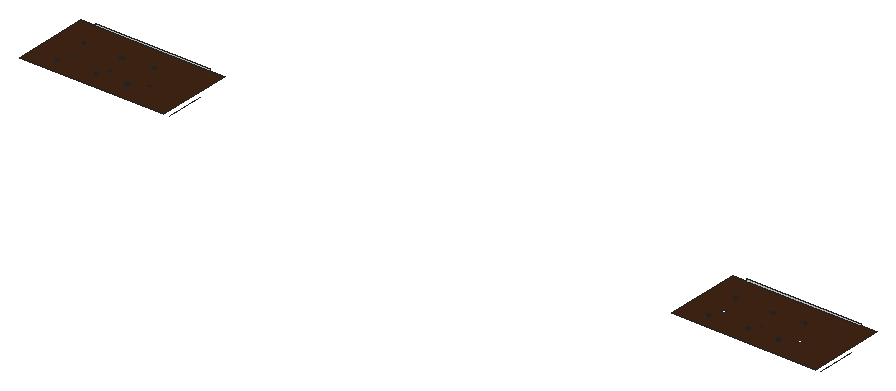
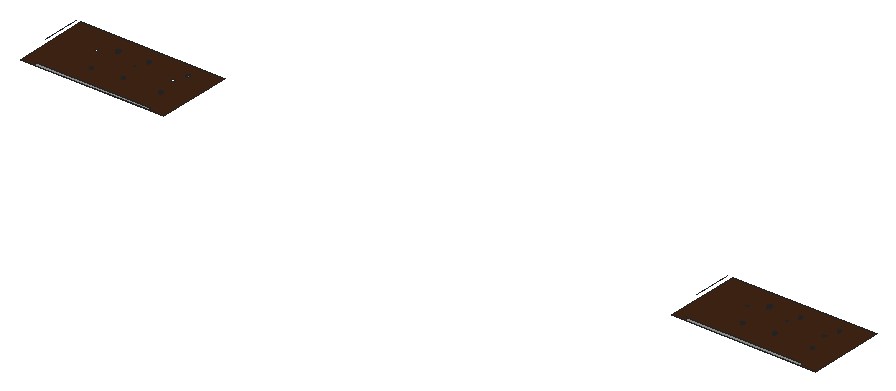
# SketchUp Ruby script. Lengths in inches.
U = 1.inch
M = Sketchup.active_model
def pt(a) = Geom::Point3d.new(a.map { |v| v * U })
def face(e, loops, mat)
  f = e.add_face(loops[0].map { |a| pt(a) })
  loops[1..].each { |l| e.add_face(l.map { |a| pt(a) }).erase! }
  f.material = f.back_material = mat if mat
  f
end
# faces: each face lists its corners as indices into pts; further lists are holes
def faces(e, pts, list, mat = nil) = list.each { |f| face(e, (f[0].is_a?(Array) ? f : [f]).map { |l| l.map { |i| pts[i] } }, mat) }
# xy, xz, yz: faces in a plane at the given z, y or x. An outline is a flat list of corners, or four numbers for a rectangle; further outlines are holes
def ring(l) = l.size == 4 ? [[l[0], l[1]], [l[2], l[1]], [l[2], l[3]], [l[0], l[3]]] : l.each_slice(2).to_a
def flat(e, list, mat, &to3) = list.each { |f| face(e, (f[0].is_a?(Array) ? f : [f]).map { |l| ring(l).map { |u, v| to3.(u, v) } }, mat) }
def xy(e, z, list, mat = nil) = flat(e, list, mat) { |x, y| [x, y, z] }
def xz(e, y, list, mat = nil) = flat(e, list, mat) { |x, z| [x, y, z] }
def yz(e, x, list, mat = nil) = flat(e, list, mat) { |y, z| [x, y, z] }
def lines(e, pts, list) = list.each { |a, b| e.add_line(pt(pts[a]), pt(pts[b])) }
# prism: a flat outline (further loops are holes) pulled along v
def prism(e, loops, v, mat = nil)
  f = face(e, loops, mat); d = Geom::Vector3d.new(v.map { |x| x * U })
  f.pushpull(f.normal.samedirection?(d) ? d.length : -d.length)
end
def box(e, o, s, mat = nil) = prism(e, [[o, [o[0] + s[0], o[1], o[2]], [o[0] + s[0], o[1] + s[1], o[2]], [o[0], o[1] + s[1], o[2]]]], [0, 0, s[2]], mat)
def at(x, y, z, deg = 0) = Geom::Transformation.translation(pt([x, y, z])) * Geom::Transformation.rotation(ORIGIN, Z_AXIS, deg.degrees)
def axes(o, x, y, z) = Geom::Transformation.new([*x, 0, *y, 0, *z, 0, *pt(o).to_a, 1])
def part(name) = M.definitions.add(name)
# library, detail: a bought-in or finely detailed component or shape, given as its bounding box
def library(name, o, s) = part(name).tap { |d| box(d.entities, o, s) }
def detail(e, o, s) = box(e.add_group.entities, o, s)
def put(e, d, t, mat = nil) = e.add_instance(d, t).tap { |i| i.material = mat if mat }
def group(e, t, mat = nil) = e.add_group.tap { |g| g.transformation = t; g.material = mat if mat }.entities
root = M.entities
M.materials.add("[Field Square Tile]").color = [211, 167, 108]
M.materials.add("[Wood Veneer 01]").color = [66, 38, 20]
xy(root,251.5,[[[1990.46,458.5,2184.6,561.05],[2030.6,492.27,2031.39,492.375,2032.13,492.68,2032.76,493.17,2033.25,493.8,2033.56,494.54,2033.66,495.33,2033.56,496.125,2033.25,496.86,2032.76,497.5,2032.13,497.98,2031.39,498.29,2030.6,498.39,2029.81,498.29,2029.07,497.98,2028.43,497.5,2027.95,496.86,2027.64,496.125,2027.54,495.33,2027.64,494.54,2027.95,493.8,2028.43,493.17,2029.07,492.68,2029.81,492.375],[2134.54,492.58,2135.25,492.68,2135.92,492.95,2136.49,493.39,2136.92,493.96,2137.2,494.62,2137.29,495.33,2137.2,496.04,2136.92,496.71,2136.49,497.28,2135.92,497.71,2135.25,497.99,2134.54,498.08,2133.83,497.99,2133.17,497.71,2132.6,497.28,2132.16,496.71,2131.89,496.04,2131.79,495.33,2131.89,494.62,2132.16,493.96,2132.6,493.39,2133.17,492.95,2133.83,492.68],[2081.97,492.77,2082.63,492.86,2083.25,493.11,2083.78,493.52,2084.19,494.05,2084.45,494.67,2084.53,495.33,2084.45,495.99,2084.19,496.61,2083.78,497.14,2083.25,497.55,2082.63,497.81,2081.97,497.89,2081.31,497.81,2080.69,497.55,2080.16,497.14,2079.75,496.61,2079.5,495.99,2079.41,495.33,2079.5,494.67,2079.75,494.05,2080.16,493.52,2080.69,493.11,2081.31,492.86],[2114.7,481.02,2115.33,481.11,2115.92,481.35,2116.42,481.74,2116.81,482.24,2117.05,482.83,2117.13,483.46,2117.05,484.09,2116.81,484.68,2116.42,485.18,2115.92,485.57,2115.33,485.8125,2114.7,485.9,2114.07,485.8125,2113.48,485.57,2112.97,485.18,2112.59,484.68,2112.34,484.09,2112.26,483.46,2112.34,482.83,2112.59,482.24,2112.97,481.74,2113.48,481.35,2114.07,481.11],[2024.3,476.64,2024.78,476.71,2025.24,476.89,2025.625,477.19,2025.92,477.58,2026.11,478.03,2026.17,478.52,2026.11,479,2025.92,479.45,2025.625,479.84,2025.24,480.14,2024.78,480.33,2024.3,480.39,2023.8125,480.33,2023.36,480.14,2022.97,479.84,2022.67,479.45,2022.49,479,2022.42,478.52,2022.49,478.03,2022.67,477.58,2022.97,477.19,2023.36,476.89,2023.8125,476.71],[2024.3,522.58,2024.78,522.64,2025.24,522.83,2025.625,523.13,2025.92,523.52,2026.11,523.97,2026.17,524.45,2026.11,524.94,2025.92,525.39,2025.625,525.78,2025.24,526.08,2024.78,526.27,2024.3,526.33,2023.8125,526.27,2023.36,526.08,2022.97,525.78,2022.67,525.39,2022.49,524.94,2022.42,524.45,2022.49,523.97,2022.67,523.52,2022.97,523.13,2023.36,522.83,2023.8125,522.64],[2074.74,522.58,2075.22,522.64,2075.67,522.83,2076.0625,523.13,2076.36,523.52,2076.55,523.97,2076.61,524.45,2076.55,524.94,2076.36,525.39,2076.0625,525.78,2075.67,526.08,2075.22,526.27,2074.74,526.33,2074.25,526.27,2073.8,526.08,2073.41,525.78,2073.11,525.39,2072.92,524.94,2072.86,524.45,2072.92,523.97,2073.11,523.52,2073.41,523.13,2073.8,522.83,2074.25,522.64],[2074.74,479.77,2075.22,479.83,2075.67,480.02,2076.0625,480.32,2076.36,480.7,2076.55,481.16,2076.61,481.64,2076.55,482.13,2076.36,482.58,2076.0625,482.97,2075.67,483.27,2075.22,483.45,2074.74,483.52,2074.25,483.45,2073.8,483.27,2073.41,482.97,2073.11,482.58,2072.92,482.13,2072.86,481.64,2072.92,481.16,2073.11,480.7,2073.41,480.32,2073.8,480.02,2074.25,479.83],[2114.7,526.75,2115.13,526.8125,2115.54,526.98,2115.89,527.25,2116.16,527.6,2116.33,528,2116.38,528.44,2116.33,528.88,2116.16,529.28,2115.89,529.63,2115.54,529.9,2115.13,530.07,2114.7,530.13,2114.26,530.07,2113.85,529.9,2113.5,529.63,2113.24,529.28,2113.07,528.88,2113.01,528.44,2113.07,528,2113.24,527.6,2113.5,527.25,2113.85,526.98,2114.26,526.8125]],[[2869.21,458.5,3063.35,561.05],[2909.35,492.27,2910.14,492.375,2910.88,492.68,2911.51,493.17,2912,493.8,2912.31,494.54,2912.41,495.33,2912.31,496.125,2912,496.86,2911.51,497.5,2910.88,497.98,2910.14,498.29,2909.35,498.39,2908.56,498.29,2907.82,497.98,2907.18,497.5,2906.7,496.86,2906.39,496.125,2906.29,495.33,2906.39,494.54,2906.7,493.8,2907.18,493.17,2907.82,492.68,2908.56,492.375],[3013.29,492.58,3014,492.68,3014.67,492.95,3015.24,493.39,3015.67,493.96,3015.95,494.62,3016.04,495.33,3015.95,496.04,3015.67,496.71,3015.24,497.28,3014.67,497.71,3014,497.99,3013.29,498.08,3012.58,497.99,3011.92,497.71,3011.35,497.28,3010.91,496.71,3010.64,496.04,3010.54,495.33,3010.64,494.62,3010.91,493.96,3011.35,493.39,3011.92,492.95,3012.58,492.68],[2960.72,492.77,2961.38,492.86,2962,493.11,2962.53,493.52,2962.94,494.05,2963.2,494.67,2963.28,495.33,2963.2,495.99,2962.94,496.61,2962.53,497.14,2962,497.55,2961.38,497.81,2960.72,497.89,2960.06,497.81,2959.44,497.55,2958.91,497.14,2958.5,496.61,2958.25,495.99,2958.16,495.33,2958.25,494.67,2958.5,494.05,2958.91,493.52,2959.44,493.11,2960.06,492.86],[2993.45,481.02,2994.08,481.11,2994.67,481.35,2995.17,481.74,2995.56,482.24,2995.8,482.83,2995.88,483.46,2995.8,484.09,2995.56,484.68,2995.17,485.18,2994.67,485.57,2994.08,485.8125,2993.45,485.9,2992.82,485.8125,2992.23,485.57,2991.72,485.18,2991.34,484.68,2991.09,484.09,2991.01,483.46,2991.09,482.83,2991.34,482.24,2991.72,481.74,2992.23,481.35,2992.82,481.11],[2903.05,522.58,2903.53,522.64,2903.99,522.83,2904.375,523.13,2904.67,523.52,2904.86,523.97,2904.92,524.45,2904.86,524.94,2904.67,525.39,2904.375,525.78,2903.99,526.08,2903.53,526.27,2903.05,526.33,2902.5625,526.27,2902.11,526.08,2901.72,525.78,2901.42,525.39,2901.24,524.94,2901.17,524.45,2901.24,523.97,2901.42,523.52,2901.72,523.13,2902.11,522.83,2902.5625,522.64],[2953.49,522.58,2953.97,522.64,2954.42,522.83,2954.8125,523.13,2955.11,523.52,2955.3,523.97,2955.36,524.45,2955.3,524.94,2955.11,525.39,2954.8125,525.78,2954.42,526.08,2953.97,526.27,2953.49,526.33,2953,526.27,2952.55,526.08,2952.16,525.78,2951.86,525.39,2951.67,524.94,2951.61,524.45,2951.67,523.97,2951.86,523.52,2952.16,523.13,2952.55,522.83,2953,522.64],[2953.49,479.77,2953.97,479.83,2954.42,480.02,2954.8125,480.32,2955.11,480.7,2955.3,481.16,2955.36,481.64,2955.3,482.13,2955.11,482.58,2954.8125,482.97,2954.42,483.27,2953.97,483.45,2953.49,483.52,2953,483.45,2952.55,483.27,2952.16,482.97,2951.86,482.58,2951.67,482.13,2951.61,481.64,2951.67,481.16,2951.86,480.7,2952.16,480.32,2952.55,480.02,2953,479.83],[2903.05,476.64,2903.53,476.71,2903.99,476.89,2904.375,477.19,2904.67,477.58,2904.86,478.03,2904.92,478.52,2904.86,479,2904.67,479.45,2904.375,479.84,2903.99,480.14,2903.53,480.33,2903.05,480.39,2902.5625,480.33,2902.11,480.14,2901.72,479.84,2901.42,479.45,2901.24,479,2901.17,478.52,2901.24,478.03,2901.42,477.58,2901.72,477.19,2902.11,476.89,2902.5625,476.71],[2993.45,526.75,2993.88,526.8125,2994.29,526.98,2994.64,527.25,2994.91,527.6,2995.08,528,2995.13,528.44,2995.08,528.88,2994.91,529.28,2994.64,529.63,2994.29,529.9,2993.88,530.07,2993.45,530.13,2993.01,530.07,2992.6,529.9,2992.25,529.63,2991.99,529.28,2991.82,528.88,2991.76,528.44,2991.82,528,2991.99,527.6,2992.25,527.25,2992.6,526.98,2993.01,526.8125]]],"[Wood Veneer 01]")
xz(root,561.05,[[2010.28,251.5,2010.34,254.5],[2010.34,251.5,2164.35,254.5],[2889.03,251.5,2889.09,254.5],[2889.09,251.5,3043.1,254.5]])
p = [[2024.3,476.64,251.5],[2023.8125,476.71,251.5],[2023.8125,476.71,252.5],[2024.3,476.64,252.5],[2024.78,476.71,251.5],[2024.78,476.71,252.5],
  [2903.05,476.64,251.5],[2902.5625,476.71,251.5],[2902.5625,476.71,252.5],[2903.05,476.64,252.5],[2903.53,476.71,251.5],[2903.53,476.71,252.5],
  [2023.36,476.89,251.5],[2023.36,476.89,252.5],[2025.24,476.89,251.5],[2025.24,476.89,252.5],[2902.11,476.89,251.5],[2902.11,476.89,252.5],
  [2903.99,476.89,251.5],[2903.99,476.89,252.5],[2022.97,477.19,251.5],[2022.97,477.19,252.5],[2025.625,477.19,251.5],[2025.625,477.19,252.5],
  [2901.72,477.19,251.5],[2901.72,477.19,252.5],[2904.375,477.19,251.5],[2904.375,477.19,252.5],[2022.67,477.58,251.5],[2022.67,477.58,252.5],
  [2025.92,477.58,251.5],[2025.92,477.58,252.5],[2901.42,477.58,251.5],[2901.42,477.58,252.5],[2904.67,477.58,251.5],[2904.67,477.58,252.5],
  [2022.49,478.03,251.5],[2022.49,478.03,252.5],[2026.11,478.03,251.5],[2026.11,478.03,252.5],[2901.24,478.03,251.5],[2901.24,478.03,252.5],
  [2904.86,478.03,251.5],[2904.86,478.03,252.5],[2022.42,478.52,251.5],[2022.42,478.52,252.5],[2026.17,478.52,251.5],[2026.17,478.52,252.5],
  [2901.17,478.52,251.5],[2901.17,478.52,252.5],[2904.92,478.52,251.5],[2904.92,478.52,252.5],[2022.49,479,251.5],[2022.49,479,252.5],
  [2026.11,479,251.5],[2026.11,479,252.5],[2901.24,479,251.5],[2901.24,479,252.5],[2904.86,479,251.5],[2904.86,479,252.5],
  [2022.67,479.45,251.5],[2022.67,479.45,252.5],[2025.92,479.45,251.5],[2025.92,479.45,252.5],[2901.42,479.45,251.5],[2901.42,479.45,252.5],
  [2904.67,479.45,251.5],[2904.67,479.45,252.5],[2022.97,479.84,251.5],[2022.97,479.84,252.5],[2025.625,479.84,251.5],[2025.625,479.84,252.5],
  [2901.72,479.84,251.5],[2901.72,479.84,252.5],[2904.375,479.84,251.5],[2904.375,479.84,252.5],[2023.36,480.14,251.5],[2023.36,480.14,252.5],
  [2025.24,480.14,251.5],[2025.24,480.14,252.5],[2074.25,479.83,251.5],[2073.8,480.02,251.5],[2073.8,480.02,252.5],[2074.25,479.83,252.5],
  [2074.74,479.77,251.5],[2074.74,479.77,252.5],[2075.22,479.83,251.5],[2075.22,479.83,252.5],[2075.67,480.02,251.5],[2075.67,480.02,252.5],
  [2902.11,480.14,251.5],[2902.11,480.14,252.5],[2903.99,480.14,251.5],[2903.99,480.14,252.5],[2953,479.83,251.5],[2952.55,480.02,251.5],
  [2952.55,480.02,252.5],[2953,479.83,252.5],[2953.49,479.77,251.5],[2953.49,479.77,252.5],[2953.97,479.83,251.5],[2953.97,479.83,252.5],
  [2954.42,480.02,251.5],[2954.42,480.02,252.5],[2073.41,480.32,251.5],[2073.41,480.32,252.5],[2076.0625,480.32,251.5],[2076.0625,480.32,252.5],
  [2952.16,480.32,251.5],[2952.16,480.32,252.5],[2954.8125,480.32,251.5],[2954.8125,480.32,252.5],[2023.8125,480.33,251.5],[2023.8125,480.33,252.5],
  [2024.78,480.33,251.5],[2024.78,480.33,252.5],[2902.5625,480.33,251.5],[2902.5625,480.33,252.5],[2903.53,480.33,251.5],[2903.53,480.33,252.5],
  [2024.3,480.39,251.5],[2024.3,480.39,252.5],[2073.11,480.7,251.5],[2073.11,480.7,252.5],[2076.36,480.7,251.5],[2076.36,480.7,252.5],
  [2903.05,480.39,251.5],[2903.05,480.39,252.5],[2951.86,480.7,251.5],[2951.86,480.7,252.5],[2955.11,480.7,251.5],[2955.11,480.7,252.5],
  [2072.92,481.16,251.5],[2072.92,481.16,252.5],[2076.55,481.16,251.5],[2076.55,481.16,252.5],[2951.67,481.16,251.5],[2951.67,481.16,252.5],
  [2955.3,481.16,251.5],[2955.3,481.16,252.5],[2114.7,481.02,251.5],[2114.07,481.11,251.5],[2114.07,481.11,252.5625],[2114.7,481.02,252.5625],
  [2115.33,481.11,251.5],[2115.33,481.11,252.5625],[2993.45,481.02,251.5],[2992.82,481.11,251.5],[2992.82,481.11,252.5625],[2993.45,481.02,252.5625],
  [2994.08,481.11,251.5],[2994.08,481.11,252.5625],[2113.48,481.35,251.5],[2113.48,481.35,252.5625],[2115.92,481.35,251.5],[2115.92,481.35,252.5625],
  [2992.23,481.35,251.5],[2992.23,481.35,252.5625],[2994.67,481.35,251.5],[2994.67,481.35,252.5625],[2072.86,481.64,251.5],[2072.86,481.64,252.5],
  [2076.61,481.64,251.5],[2076.61,481.64,252.5],[2951.61,481.64,251.5],[2951.61,481.64,252.5],[2955.36,481.64,251.5],[2955.36,481.64,252.5],
  [2112.97,481.74,251.5],[2112.97,481.74,252.5625],[2116.42,481.74,251.5],[2116.42,481.74,252.5625],[2991.72,481.74,251.5],[2991.72,481.74,252.5625],
  [2995.17,481.74,251.5],[2995.17,481.74,252.5625],[2072.92,482.13,251.5],[2072.92,482.13,252.5],[2076.55,482.13,251.5],[2076.55,482.13,252.5],
  [2951.67,482.13,251.5],[2951.67,482.13,252.5],[2955.3,482.13,251.5],[2955.3,482.13,252.5],[2112.59,482.24,251.5],[2112.59,482.24,252.5625],
  [2116.81,482.24,251.5],[2116.81,482.24,252.5625],[2991.34,482.24,251.5],[2991.34,482.24,252.5625],[2995.56,482.24,251.5],[2995.56,482.24,252.5625],
  [2073.11,482.58,251.5],[2073.11,482.58,252.5],[2076.36,482.58,251.5],[2076.36,482.58,252.5],[2951.86,482.58,251.5],[2951.86,482.58,252.5],
  [2955.11,482.58,251.5],[2955.11,482.58,252.5],[2112.34,482.83,251.5],[2112.34,482.83,252.5625],[2117.05,482.83,251.5],[2117.05,482.83,252.5625],
  [2991.09,482.83,251.5],[2991.09,482.83,252.5625],[2995.8,482.83,251.5],[2995.8,482.83,252.5625],[2073.41,482.97,251.5],[2073.41,482.97,252.5],
  [2076.0625,482.97,251.5],[2076.0625,482.97,252.5],[2952.16,482.97,251.5],[2952.16,482.97,252.5],[2954.8125,482.97,251.5],[2954.8125,482.97,252.5],
  [2112.26,483.46,251.5],[2112.26,483.46,252.5625],[2117.13,483.46,251.5],[2117.13,483.46,252.5625],[2991.01,483.46,251.5],[2991.01,483.46,252.5625],
  [2995.88,483.46,251.5],[2995.88,483.46,252.5625],[2073.8,483.27,251.5],[2073.8,483.27,252.5],[2075.67,483.27,251.5],[2075.67,483.27,252.5],
  [2952.55,483.27,251.5],[2952.55,483.27,252.5],[2954.42,483.27,251.5],[2954.42,483.27,252.5],[2074.25,483.45,251.5],[2074.25,483.45,252.5],
  [2075.22,483.45,251.5],[2075.22,483.45,252.5],[2953,483.45,251.5],[2953,483.45,252.5],[2953.97,483.45,251.5],[2953.97,483.45,252.5],
  [2074.74,483.52,251.5],[2074.74,483.52,252.5],[2112.34,484.09,251.5],[2112.34,484.09,252.5625],[2117.05,484.09,251.5],[2117.05,484.09,252.5625],
  [2953.49,483.52,251.5],[2953.49,483.52,252.5],[2991.09,484.09,251.5],[2991.09,484.09,252.5625],[2995.8,484.09,251.5],[2995.8,484.09,252.5625],
  [2112.59,484.68,251.5],[2112.59,484.68,252.5625],[2116.81,484.68,251.5],[2116.81,484.68,252.5625],[2991.34,484.68,251.5],[2991.34,484.68,252.5625],
  [2995.56,484.68,251.5],[2995.56,484.68,252.5625],[2112.97,485.18,251.5],[2112.97,485.18,252.5625],[2116.42,485.18,251.5],[2116.42,485.18,252.5625],
  [2991.72,485.18,251.5],[2991.72,485.18,252.5625],[2995.17,485.18,251.5],[2995.17,485.18,252.5625],[2113.48,485.57,251.5],[2113.48,485.57,252.5625],
  [2115.92,485.57,251.5],[2115.92,485.57,252.5625],[2992.23,485.57,251.5],[2992.23,485.57,252.5625],[2994.67,485.57,251.5],[2994.67,485.57,252.5625],
  [2114.07,485.8125,251.5],[2114.07,485.8125,252.5625],[2115.33,485.8125,251.5],[2115.33,485.8125,252.5625],[2992.82,485.8125,251.5],[2992.82,485.8125,252.5625],
  [2994.08,485.8125,251.5],[2994.08,485.8125,252.5625],[2114.7,485.9,251.5],[2114.7,485.9,252.5625],[2993.45,485.9,251.5],[2993.45,485.9,252.5625],
  [2023.8125,522.64,251.5],[2023.36,522.83,251.5],[2023.36,522.83,252.5],[2023.8125,522.64,252.5],[2024.3,522.58,251.5],[2024.3,522.58,252.5],
  [2024.78,522.64,251.5],[2024.78,522.64,252.5],[2025.24,522.83,251.5],[2025.24,522.83,252.5],[2074.25,522.64,251.5],[2073.8,522.83,251.5],
  [2073.8,522.83,252.5],[2074.25,522.64,252.5],[2074.74,522.58,251.5],[2074.74,522.58,252.5],[2075.22,522.64,251.5],[2075.22,522.64,252.5],
  [2075.67,522.83,251.5],[2075.67,522.83,252.5],[2902.5625,522.64,251.5],[2902.11,522.83,251.5],[2902.11,522.83,252.5],[2902.5625,522.64,252.5],
  [2903.05,522.58,251.5],[2903.05,522.58,252.5],[2903.53,522.64,251.5],[2903.53,522.64,252.5],[2903.99,522.83,251.5],[2903.99,522.83,252.5],
  [2953,522.64,251.5],[2952.55,522.83,251.5],[2952.55,522.83,252.5],[2953,522.64,252.5],[2953.49,522.58,251.5],[2953.49,522.58,252.5],
  [2953.97,522.64,251.5],[2953.97,522.64,252.5],[2954.42,522.83,251.5],[2954.42,522.83,252.5],[2022.97,523.13,251.5],[2022.97,523.13,252.5],
  [2025.625,523.13,251.5],[2025.625,523.13,252.5],[2073.41,523.13,251.5],[2073.41,523.13,252.5],[2076.0625,523.13,251.5],[2076.0625,523.13,252.5],
  [2901.72,523.13,251.5],[2901.72,523.13,252.5],[2904.375,523.13,251.5],[2904.375,523.13,252.5],[2952.16,523.13,251.5],[2952.16,523.13,252.5],
  [2954.8125,523.13,251.5],[2954.8125,523.13,252.5],[2022.67,523.52,251.5],[2022.67,523.52,252.5],[2025.92,523.52,251.5],[2025.92,523.52,252.5],
  [2073.11,523.52,251.5],[2073.11,523.52,252.5],[2076.36,523.52,251.5],[2076.36,523.52,252.5],[2901.42,523.52,251.5],[2901.42,523.52,252.5],
  [2904.67,523.52,251.5],[2904.67,523.52,252.5],[2951.86,523.52,251.5],[2951.86,523.52,252.5],[2955.11,523.52,251.5],[2955.11,523.52,252.5],
  [2022.49,523.97,251.5],[2022.49,523.97,252.5],[2026.11,523.97,251.5],[2026.11,523.97,252.5],[2072.92,523.97,251.5],[2072.92,523.97,252.5],
  [2076.55,523.97,251.5],[2076.55,523.97,252.5],[2901.24,523.97,251.5],[2901.24,523.97,252.5],[2904.86,523.97,251.5],[2904.86,523.97,252.5],
  [2951.67,523.97,251.5],[2951.67,523.97,252.5],[2955.3,523.97,251.5],[2955.3,523.97,252.5],[2022.42,524.45,251.5],[2022.42,524.45,252.5],
  [2026.17,524.45,251.5],[2026.17,524.45,252.5],[2072.86,524.45,251.5],[2072.86,524.45,252.5],[2076.61,524.45,251.5],[2076.61,524.45,252.5],
  [2901.17,524.45,251.5],[2901.17,524.45,252.5],[2904.92,524.45,251.5],[2904.92,524.45,252.5],[2951.61,524.45,251.5],[2951.61,524.45,252.5],
  [2955.36,524.45,251.5],[2955.36,524.45,252.5],[2022.49,524.94,251.5],[2022.49,524.94,252.5],[2026.11,524.94,251.5],[2026.11,524.94,252.5],
  [2072.92,524.94,251.5],[2072.92,524.94,252.5],[2076.55,524.94,251.5],[2076.55,524.94,252.5],[2901.24,524.94,251.5],[2901.24,524.94,252.5],
  [2904.86,524.94,251.5],[2904.86,524.94,252.5],[2951.67,524.94,251.5],[2951.67,524.94,252.5],[2955.3,524.94,251.5],[2955.3,524.94,252.5],
  [2022.67,525.39,251.5],[2022.67,525.39,252.5],[2025.92,525.39,251.5],[2025.92,525.39,252.5],[2073.11,525.39,251.5],[2073.11,525.39,252.5],
  [2076.36,525.39,251.5],[2076.36,525.39,252.5],[2901.42,525.39,251.5],[2901.42,525.39,252.5],[2904.67,525.39,251.5],[2904.67,525.39,252.5],
  [2951.86,525.39,251.5],[2951.86,525.39,252.5],[2955.11,525.39,251.5],[2955.11,525.39,252.5],[2022.97,525.78,251.5],[2022.97,525.78,252.5],
  [2025.625,525.78,251.5],[2025.625,525.78,252.5],[2073.41,525.78,251.5],[2073.41,525.78,252.5],[2076.0625,525.78,251.5],[2076.0625,525.78,252.5],
  [2901.72,525.78,251.5],[2901.72,525.78,252.5],[2904.375,525.78,251.5],[2904.375,525.78,252.5],[2952.16,525.78,251.5],[2952.16,525.78,252.5],
  [2954.8125,525.78,251.5],[2954.8125,525.78,252.5],[2023.36,526.08,251.5],[2023.36,526.08,252.5],[2025.24,526.08,251.5],[2025.24,526.08,252.5],
  [2073.8,526.08,251.5],[2073.8,526.08,252.5],[2075.67,526.08,251.5],[2075.67,526.08,252.5],[2902.11,526.08,251.5],[2902.11,526.08,252.5],
  [2903.99,526.08,251.5],[2903.99,526.08,252.5],[2952.55,526.08,251.5],[2952.55,526.08,252.5],[2954.42,526.08,251.5],[2954.42,526.08,252.5],
  [2023.8125,526.27,251.5],[2023.8125,526.27,252.5],[2024.78,526.27,251.5],[2024.78,526.27,252.5],[2074.25,526.27,251.5],[2074.25,526.27,252.5],
  [2075.22,526.27,251.5],[2075.22,526.27,252.5],[2902.5625,526.27,251.5],[2902.5625,526.27,252.5],[2903.53,526.27,251.5],[2903.53,526.27,252.5],
  [2953,526.27,251.5],[2953,526.27,252.5],[2953.97,526.27,251.5],[2953.97,526.27,252.5],[2024.3,526.33,251.5],[2024.3,526.33,252.5],
  [2074.74,526.33,251.5],[2074.74,526.33,252.5],[2903.05,526.33,251.5],[2903.05,526.33,252.5],[2953.49,526.33,251.5],[2953.49,526.33,252.5],
  [2114.26,526.8125,251.5],[2113.85,526.98,251.5],[2113.85,526.98,252.4375],[2114.26,526.8125,252.4375],[2114.7,526.75,251.5],[2114.7,526.75,252.4375],
  [2115.13,526.8125,251.5],[2115.13,526.8125,252.4375],[2115.54,526.98,251.5],[2115.54,526.98,252.4375],[2993.01,526.8125,251.5],[2992.6,526.98,251.5],
  [2992.6,526.98,252.4375],[2993.01,526.8125,252.4375],[2993.45,526.75,251.5],[2993.45,526.75,252.4375],[2993.88,526.8125,251.5],[2993.88,526.8125,252.4375],
  [2994.29,526.98,251.5],[2994.29,526.98,252.4375],[2113.5,527.25,251.5],[2113.5,527.25,252.4375],[2115.89,527.25,251.5],[2115.89,527.25,252.4375],
  [2992.25,527.25,251.5],[2992.25,527.25,252.4375],[2994.64,527.25,251.5],[2994.64,527.25,252.4375],[2113.24,527.6,251.5],[2113.24,527.6,252.4375],
  [2116.16,527.6,251.5],[2116.16,527.6,252.4375],[2991.99,527.6,251.5],[2991.99,527.6,252.4375],[2994.91,527.6,251.5],[2994.91,527.6,252.4375],
  [2113.07,528,251.5],[2113.07,528,252.4375],[2116.33,528,251.5],[2116.33,528,252.4375],[2991.82,528,251.5],[2991.82,528,252.4375],
  [2995.08,528,251.5],[2995.08,528,252.4375],[2113.01,528.44,251.5],[2113.01,528.44,252.4375],[2116.38,528.44,251.5],[2116.38,528.44,252.4375],
  [2991.76,528.44,251.5],[2991.76,528.44,252.4375],[2995.13,528.44,251.5],[2995.13,528.44,252.4375],[2113.07,528.88,251.5],[2113.07,528.88,252.4375],
  [2116.33,528.88,251.5],[2116.33,528.88,252.4375],[2991.82,528.88,251.5],[2991.82,528.88,252.4375],[2995.08,528.88,251.5],[2995.08,528.88,252.4375],
  [2113.24,529.28,251.5],[2113.24,529.28,252.4375],[2116.16,529.28,251.5],[2116.16,529.28,252.4375],[2991.99,529.28,251.5],[2991.99,529.28,252.4375],
  [2994.91,529.28,251.5],[2994.91,529.28,252.4375],[2113.5,529.63,251.5],[2113.5,529.63,252.4375],[2115.89,529.63,251.5],[2115.89,529.63,252.4375],
  [2992.25,529.63,251.5],[2992.25,529.63,252.4375],[2994.64,529.63,251.5],[2994.64,529.63,252.4375],[2113.85,529.9,251.5],[2113.85,529.9,252.4375],
  [2115.54,529.9,251.5],[2115.54,529.9,252.4375],[2992.6,529.9,251.5],[2992.6,529.9,252.4375],[2994.29,529.9,251.5],[2994.29,529.9,252.4375],
  [2114.26,530.07,251.5],[2114.26,530.07,252.4375],[2115.13,530.07,251.5],[2115.13,530.07,252.4375],[2993.01,530.07,251.5],[2993.01,530.07,252.4375],
  [2993.88,530.07,251.5],[2993.88,530.07,252.4375],[2114.7,530.13,251.5],[2114.7,530.13,252.4375],[2993.45,530.13,251.5],[2993.45,530.13,252.4375],
  [2191.47,511.08,251.5],[2191.47,458.5,251.5],[3070.22,511.08,251.5],[3070.22,458.5,251.5]]
faces(root,p,[[0,1,2,3],[4,0,3,5],[6,7,8,9],[10,6,9,11],[1,12,13,2],[14,4,5,15],[7,16,17,8],[18,10,11,19],
  [12,20,21,13],[22,14,15,23],[16,24,25,17],[26,18,19,27],[20,28,29,21],[30,22,23,31],[24,32,33,25],[34,26,27,35],
  [28,36,37,29],[38,30,31,39],[32,40,41,33],[42,34,35,43],[36,44,45,37],[46,38,39,47],[40,48,49,41],[50,42,43,51],
  [44,52,53,45],[54,46,47,55],[48,56,57,49],[58,50,51,59],[52,60,61,53],[62,54,55,63],[56,64,65,57],[66,58,59,67],
  [60,68,69,61],[70,62,63,71],[64,72,73,65],[74,66,67,75],[68,76,77,69],[78,70,71,79],[80,81,82,83],[84,80,83,85],
  [86,84,85,87],[88,86,87,89],[72,90,91,73],[92,74,75,93],[94,95,96,97],[98,94,97,99],[100,98,99,101],[102,100,101,103],
  [81,104,105,82],[106,88,89,107],[95,108,109,96],[110,102,103,111],[76,112,113,77],[114,78,79,115],[90,116,117,91],[118,92,93,119],
  [112,120,121,113],[120,114,115,121],[104,122,123,105],[124,106,107,125],[116,126,127,117],[126,118,119,127],[108,128,129,109],[130,110,111,131],
  [122,132,133,123],[134,124,125,135],[128,136,137,129],[138,130,131,139],[140,141,142,143],[144,140,143,145],[146,147,148,149],[150,146,149,151],
  [141,152,153,142],[154,144,145,155],[147,156,157,148],[158,150,151,159],[132,160,161,133],[162,134,135,163],[136,164,165,137],[166,138,139,167],
  [152,168,169,153],[170,154,155,171],[156,172,173,157],[174,158,159,175],[160,176,177,161],[178,162,163,179],[164,180,181,165],[182,166,167,183],
  [168,184,185,169],[186,170,171,187],[172,188,189,173],[190,174,175,191],[176,192,193,177],[194,178,179,195],[180,196,197,181],[198,182,183,199],
  [184,200,201,185],[202,186,187,203],[188,204,205,189],[206,190,191,207],[192,208,209,193],[210,194,195,211],[196,212,213,197],[214,198,199,215],
  [200,216,217,201],[218,202,203,219],[204,220,221,205],[222,206,207,223],[208,224,225,209],[226,210,211,227],[212,228,229,213],[230,214,215,231],
  [224,232,233,225],[234,226,227,235],[228,236,237,229],[238,230,231,239],[232,240,241,233],[240,234,235,241],[216,242,243,217],[244,218,219,245],
  [236,246,247,237],[246,238,239,247],[220,248,249,221],[250,222,223,251],[242,252,253,243],[254,244,245,255],[248,256,257,249],[258,250,251,259],
  [252,260,261,253],[262,254,255,263],[256,264,265,257],[266,258,259,267],[260,268,269,261],[270,262,263,271],[264,272,273,265],[274,266,267,275],
  [268,276,277,269],[278,270,271,279],[272,280,281,273],[282,274,275,283],[276,284,285,277],[284,278,279,285],[280,286,287,281],[286,282,283,287],
  [288,289,290,291],[292,288,291,293],[294,292,293,295],[296,294,295,297],[298,299,300,301],[302,298,301,303],[304,302,303,305],[306,304,305,307],
  [308,309,310,311],[312,308,311,313],[314,312,313,315],[316,314,315,317],[318,319,320,321],[322,318,321,323],[324,322,323,325],[326,324,325,327],
  [289,328,329,290],[330,296,297,331],[299,332,333,300],[334,306,307,335],[309,336,337,310],[338,316,317,339],[319,340,341,320],[342,326,327,343],
  [328,344,345,329],[346,330,331,347],[332,348,349,333],[350,334,335,351],[336,352,353,337],[354,338,339,355],[340,356,357,341],[358,342,343,359],
  [344,360,361,345],[362,346,347,363],[348,364,365,349],[366,350,351,367],[352,368,369,353],[370,354,355,371],[356,372,373,357],[374,358,359,375],
  [360,376,377,361],[378,362,363,379],[364,380,381,365],[382,366,367,383],[368,384,385,369],[386,370,371,387],[372,388,389,373],[390,374,375,391],
  [376,392,393,377],[394,378,379,395],[380,396,397,381],[398,382,383,399],[384,400,401,385],[402,386,387,403],[388,404,405,389],[406,390,391,407],
  [392,408,409,393],[410,394,395,411],[396,412,413,397],[414,398,399,415],[400,416,417,401],[418,402,403,419],[404,420,421,405],[422,406,407,423],
  [408,424,425,409],[426,410,411,427],[412,428,429,413],[430,414,415,431],[416,432,433,417],[434,418,419,435],[420,436,437,421],[438,422,423,439],
  [424,440,441,425],[442,426,427,443],[428,444,445,429],[446,430,431,447],[432,448,449,433],[450,434,435,451],[436,452,453,437],[454,438,439,455],
  [440,456,457,441],[458,442,443,459],[444,460,461,445],[462,446,447,463],[448,464,465,449],[466,450,451,467],[452,468,469,453],[470,454,455,471],
  [456,472,473,457],[472,458,459,473],[460,474,475,461],[474,462,463,475],[464,476,477,465],[476,466,467,477],[468,478,479,469],[478,470,471,479],
  [480,481,482,483],[484,480,483,485],[486,484,485,487],[488,486,487,489],[490,491,492,493],[494,490,493,495],[496,494,495,497],[498,496,497,499],
  [481,500,501,482],[502,488,489,503],[491,504,505,492],[506,498,499,507],[500,508,509,501],[510,502,503,511],[504,512,513,505],[514,506,507,515],
  [508,516,517,509],[518,510,511,519],[512,520,521,513],[522,514,515,523],[516,524,525,517],[526,518,519,527],[520,528,529,521],[530,522,523,531],
  [524,532,533,525],[534,526,527,535],[528,536,537,529],[538,530,531,539],[532,540,541,533],[542,534,535,543],[536,544,545,537],[546,538,539,547],
  [540,548,549,541],[550,542,543,551],[544,552,553,545],[554,546,547,555],[548,556,557,549],[558,550,551,559],[552,560,561,553],[562,554,555,563],
  [556,564,565,557],[566,558,559,567],[560,568,569,561],[570,562,563,571],[564,572,573,565],[572,566,567,573],[568,574,575,569],[574,570,571,575]],"[Field Square Tile]")
lines(root,p,[[576,577],[578,579]])
